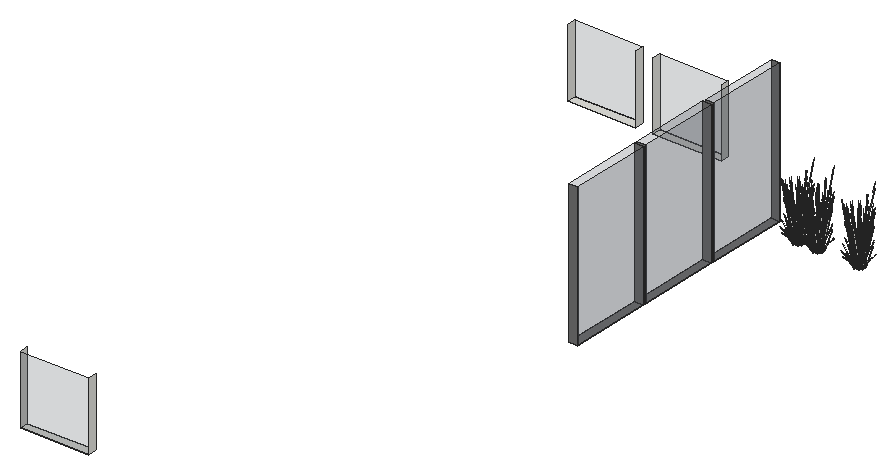
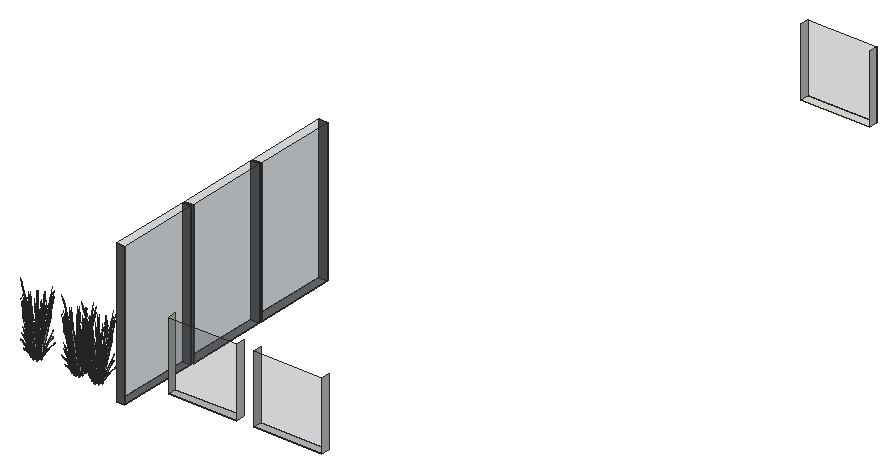
# SketchUp Ruby script. Lengths in inches.
U = 1.inch
M = Sketchup.active_model
def pt(a) = Geom::Point3d.new(a.map { |v| v * U })
def face(e, loops, mat)
  f = e.add_face(loops[0].map { |a| pt(a) })
  loops[1..].each { |l| e.add_face(l.map { |a| pt(a) }).erase! }
  f.material = f.back_material = mat if mat
  f
end
# faces: each face lists its corners as indices into pts; further lists are holes
def faces(e, pts, list, mat = nil) = list.each { |f| face(e, (f[0].is_a?(Array) ? f : [f]).map { |l| l.map { |i| pts[i] } }, mat) }
# xy, xz, yz: faces in a plane at the given z, y or x. An outline is a flat list of corners, or four numbers for a rectangle; further outlines are holes
def ring(l) = l.size == 4 ? [[l[0], l[1]], [l[2], l[1]], [l[2], l[3]], [l[0], l[3]]] : l.each_slice(2).to_a
def flat(e, list, mat, &to3) = list.each { |f| face(e, (f[0].is_a?(Array) ? f : [f]).map { |l| ring(l).map { |u, v| to3.(u, v) } }, mat) }
def xy(e, z, list, mat = nil) = flat(e, list, mat) { |x, y| [x, y, z] }
def xz(e, y, list, mat = nil) = flat(e, list, mat) { |x, z| [x, y, z] }
def yz(e, x, list, mat = nil) = flat(e, list, mat) { |y, z| [x, y, z] }
def lines(e, pts, list) = list.each { |a, b| e.add_line(pt(pts[a]), pt(pts[b])) }
# prism: a flat outline (further loops are holes) pulled along v
def prism(e, loops, v, mat = nil)
  f = face(e, loops, mat); d = Geom::Vector3d.new(v.map { |x| x * U })
  f.pushpull(f.normal.samedirection?(d) ? d.length : -d.length)
end
def box(e, o, s, mat = nil) = prism(e, [[o, [o[0] + s[0], o[1], o[2]], [o[0] + s[0], o[1] + s[1], o[2]], [o[0], o[1] + s[1], o[2]]]], [0, 0, s[2]], mat)
def at(x, y, z, deg = 0) = Geom::Transformation.translation(pt([x, y, z])) * Geom::Transformation.rotation(ORIGIN, Z_AXIS, deg.degrees)
def axes(o, x, y, z) = Geom::Transformation.new([*x, 0, *y, 0, *z, 0, *pt(o).to_a, 1])
def part(name) = M.definitions.add(name)
# library, detail: a bought-in or finely detailed component or shape, given as its bounding box
def library(name, o, s) = part(name).tap { |d| box(d.entities, o, s) }
def detail(e, o, s) = box(e.add_group.entities, o, s)
def put(e, d, t, mat = nil) = e.add_instance(d, t).tap { |i| i.material = mat if mat }
def group(e, t, mat = nil) = e.add_group.tap { |g| g.transformation = t; g.material = mat if mat }.entities
root = M.entities
M.materials.add("Glass_Basic_01").color = [105, 113, 122]
M.materials["Glass_Basic_01"].alpha = 0.25
M.materials.add("LightPink_Translucent").color = [144, 107, 117]
M.materials["LightPink_Translucent"].alpha = 0.75
M.materials.add("M06_Steel_Smoke").color = [114, 114, 114]
c1 = part("blade")
p = [[2.15,0.21,22],[0,0.17,0],[0.09,0.45,0],[2.18,0.31,22],[2.29,0.31,22],[0.38,0.45,0],
  [2.48,0.24,33],[2.49,0.24,33],[2.48,0.22,33]]
faces(c1.entities,p,[[0,1,2,3],[4,5,2,3],[6,3,4,7],[8,0,3,6]])
c2 = part("seeds")
p = [[0.3,-0.1,1.38],[-0.01,-0.03,1.59],[-0.01,-0.03,0.03],[0.14,-0.07,-0.07],[0.29,-0.03,3],[0.15,0.01,3.11]]
faces(c2.entities,p,[[0,1,2,3],[1,0,4,5]],"LightPink_Translucent")
c3 = part("blade with seeds")
put(c3.entities,c1,at(0,0,0))
put(c3.entities,c2,axes([2.4,0.25,30.99],[1.5799,-0.05474,1.17369],[-0.12525,1.92788,0.29478],[-0.07173,-0.02425,1.56792]))
xy(root,655,[[204,295,210,353],[204,355,210,413],[204,415,210,473]],"M06_Steel_Smoke")
xy(root,677.98,[[54,0,102,6]])
xy(root,678,[[60,474,108,480],[120,474,168,480]])
xz(root,0,[[54,677.98,102,725.98]],"Glass_Basic_01")
xz(root,295,[[204,655,210,755]],"M06_Steel_Smoke")
xz(root,353,[[204,655,210,755]],"M06_Steel_Smoke")
xz(root,355,[[204,655,210,755]],"M06_Steel_Smoke")
xz(root,413,[[204,655,210,755]],"M06_Steel_Smoke")
xz(root,415,[[204,655,210,755]],"M06_Steel_Smoke")
xz(root,473,[[204,655,210,755]],"M06_Steel_Smoke")
xz(root,480,[[60,678,108,726],[120,678,168,726]],"Glass_Basic_01")
yz(root,54,[[0,677.98,6,725.98]])
yz(root,60,[[474,678,480,726]])
yz(root,102,[[0,677.98,6,725.98]])
yz(root,108,[[474,678,480,726]])
yz(root,120,[[474,678,480,726]])
yz(root,168,[[474,678,480,726]])
yz(root,204,[[295,655,353,755],[355,655,413,755],[415,655,473,755]],"Glass_Basic_01")
yz(root,210,[[295,655,353,755],[355,655,413,755],[415,655,473,755]],"Glass_Basic_01")
put(root,c3,axes([234.23,462.43,655.03],[0.0269,-0.54769,-0.1216],[0.50939,0.01497,-0.67495],[0.19618,0.03804,1.02557]))
put(root,c3,axes([230.42,460.32,655.03],[0.25281,0.48765,-0.1216],[-0.44869,0.23964,-0.67495],[-0.18908,0.06434,1.02557]))
put(root,c3,axes([234.18,459.26,655.03],[-0.55221,-0.02668,-0.1216],[0.01509,-0.50521,-0.67495],[0.03836,-0.19458,1.02557]))
put(root,c3,axes([234.8,461.41,655.03],[-0.25281,-0.48765,-0.1216],[0.44869,-0.23964,-0.67495],[0.18908,-0.06434,1.02557]))
put(root,c3,axes([232.0625,463.04,655.03],[0.49168,-0.25073,-0.1216],[0.24162,0.44501,-0.67495],[0.06487,0.18753,1.02557]))
put(root,c3,axes([230.99,459.3125,655.03],[-0.0269,0.54769,-0.1216],[-0.50939,-0.01497,-0.67495],[-0.19618,-0.03804,1.02557]))
put(root,c3,axes([233.23,463.02,655.03],[0.2994,-0.46097,-0.1216],[0.43359,0.26557,-0.67495],[0.15072,0.13024,1.02557]))
put(root,c3,axes([230.44,461.48,655.03],[0.46478,0.29695,-0.1216],[-0.26776,0.43004,-0.67495],[-0.13131,0.14949,1.02557]))
put(root,c3,axes([233.16,458.7,655.03],[-0.49168,0.25073,-0.1216],[-0.24162,-0.44501,-0.67495],[-0.06487,-0.18753,1.02557]))
put(root,c3,axes([234.78,460.25,655.03],[-0.46478,-0.29695,-0.1216],[0.26776,-0.43004,-0.67495],[0.13131,-0.14949,1.02557]))
put(root,c3,axes([248.12,462.43,655.03],[0.0269,-0.54769,-0.1216],[0.50939,0.01497,-0.67495],[0.19618,0.03804,1.02557]))
put(root,c3,axes([244.31,460.32,655.03],[0.25281,0.48765,-0.1216],[-0.44869,0.23964,-0.67495],[-0.18908,0.06434,1.02557]))
put(root,c3,axes([248.07,459.26,655.03],[-0.55221,-0.02668,-0.1216],[0.01509,-0.50521,-0.67495],[0.03836,-0.19458,1.02557]))
put(root,c3,axes([248.6875,461.41,655.03],[-0.25281,-0.48765,-0.1216],[0.44869,-0.23964,-0.67495],[0.18908,-0.06434,1.02557]))
put(root,c3,axes([245.95,463.04,655.03],[0.49168,-0.25073,-0.1216],[0.24162,0.44501,-0.67495],[0.06487,0.18753,1.02557]))
put(root,c3,axes([244.88,459.3125,655.03],[-0.0269,0.54769,-0.1216],[-0.50939,-0.01497,-0.67495],[-0.19618,-0.03804,1.02557]))
put(root,c3,axes([247.12,463.02,655.03],[0.2994,-0.46097,-0.1216],[0.43359,0.26557,-0.67495],[0.15072,0.13024,1.02557]))
put(root,c3,axes([244.33,461.48,655.03],[0.46478,0.29695,-0.1216],[-0.26776,0.43004,-0.67495],[-0.13131,0.14949,1.02557]))
put(root,c3,axes([247.05,458.7,655.03],[-0.49168,0.25073,-0.1216],[-0.24162,-0.44501,-0.67495],[-0.06487,-0.18753,1.02557]))
put(root,c3,axes([248.67,460.25,655.03],[-0.46478,-0.29695,-0.1216],[0.26776,-0.43004,-0.67495],[0.13131,-0.14949,1.02557]))
put(root,c3,axes([277.23,462.43,655.03],[0.0269,-0.54769,-0.1216],[0.50939,0.01497,-0.67495],[0.19618,0.03804,1.02557]))
put(root,c3,axes([273.42,460.32,655.03],[0.25281,0.48765,-0.1216],[-0.44869,0.23964,-0.67495],[-0.18908,0.06434,1.02557]))
put(root,c3,axes([277.18,459.26,655.03],[-0.55221,-0.02668,-0.1216],[0.01509,-0.50521,-0.67495],[0.03836,-0.19458,1.02557]))
put(root,c3,axes([277.8,461.41,655.03],[-0.25281,-0.48765,-0.1216],[0.44869,-0.23964,-0.67495],[0.18908,-0.06434,1.02557]))
put(root,c3,axes([275.0625,463.04,655.03],[0.49168,-0.25073,-0.1216],[0.24162,0.44501,-0.67495],[0.06487,0.18753,1.02557]))
put(root,c3,axes([273.99,459.3125,655.03],[-0.0269,0.54769,-0.1216],[-0.50939,-0.01497,-0.67495],[-0.19618,-0.03804,1.02557]))
put(root,c3,axes([276.23,463.02,655.03],[0.2994,-0.46097,-0.1216],[0.43359,0.26557,-0.67495],[0.15072,0.13024,1.02557]))
put(root,c3,axes([273.44,461.48,655.03],[0.46478,0.29695,-0.1216],[-0.26776,0.43004,-0.67495],[-0.13131,0.14949,1.02557]))
put(root,c3,axes([276.16,458.7,655.03],[-0.49168,0.25073,-0.1216],[-0.24162,-0.44501,-0.67495],[-0.06487,-0.18753,1.02557]))
put(root,c3,axes([277.78,460.25,655.03],[-0.46478,-0.29695,-0.1216],[0.26776,-0.43004,-0.67495],[0.13131,-0.14949,1.02557]))
put(root,c3,axes([233.57,460.3,654.47],[-0.43417,-0.27982,1.38283],[0.45844,-0.43566,0.59665],[0.14008,0.26255,1.33663]))
put(root,c3,axes([247.46,460.3,654.47],[-0.43417,-0.27982,1.38283],[0.45844,-0.43566,0.59665],[0.14008,0.26255,1.33663]))
put(root,c3,axes([276.57,460.3,654.47],[-0.43417,-0.27982,1.38283],[0.45844,-0.43566,0.59665],[0.14008,0.26255,1.33663]))
put(root,c3,axes([229.89,460.8125,654.72],[-0.08205,0.06992,1.74944],[0.00698,0.51086,-0.27667],[-0.18807,0.06644,0.14031]))
put(root,c3,axes([236.18,460.65,654.72],[0.06972,-0.08203,1.74944],[-0.08924,-0.50318,-0.27667],[0.17494,-0.0954,0.14031]))
put(root,c3,axes([234.68,462.1,654.72],[0.10779,-0.00911,1.74944],[0.29564,-0.41839,-0.27667],[0.19172,0.05523,0.14031]))
put(root,c3,axes([234.68,458.46,654.72],[-0.00485,-0.10718,1.74944],[-0.40965,-0.30977,-0.27667],[0.06333,-0.18778,0.14031]))
put(root,c3,axes([229.91,462.72,654.72],[-0.01249,0.10657,1.74944],[0.35444,0.37075,-0.27667],[-0.09279,0.17532,0.14031]))
put(root,c3,axes([231.95,464.04,654.72],[0.06369,0.08672,1.74944],[0.51399,0.03407,-0.27667],[0.05169,0.19126,0.14031]))
put(root,c3,axes([232.38,457.53,654.72],[-0.07685,-0.07551,1.74944],[-0.51287,0.04787,-0.27667],[-0.08185,-0.1806,0.14031]))
put(root,c3,axes([230.7,458.36,654.72],[-0.10811,-0.0038,1.74944],[-0.34418,0.38014,-0.27667],[-0.18364,-0.07767,0.14031]))
put(root,c3,axes([243.78,460.8125,654.72],[-0.08205,0.06992,1.74944],[0.00698,0.51086,-0.27667],[-0.18807,0.06644,0.14031]))
put(root,c3,axes([250.0625,460.65,654.72],[0.06972,-0.08203,1.74944],[-0.08924,-0.50318,-0.27667],[0.17494,-0.0954,0.14031]))
put(root,c3,axes([248.5625,462.1,654.72],[0.10779,-0.00911,1.74944],[0.29564,-0.41839,-0.27667],[0.19172,0.05523,0.14031]))
put(root,c3,axes([248.57,458.46,654.72],[-0.00485,-0.10718,1.74944],[-0.40965,-0.30977,-0.27667],[0.06333,-0.18778,0.14031]))
put(root,c3,axes([243.8,462.72,654.72],[-0.01249,0.10657,1.74944],[0.35444,0.37075,-0.27667],[-0.09279,0.17532,0.14031]))
put(root,c3,axes([245.83,464.04,654.72],[0.06369,0.08672,1.74944],[0.51399,0.03407,-0.27667],[0.05169,0.19126,0.14031]))
put(root,c3,axes([246.27,457.53,654.72],[-0.07685,-0.07551,1.74944],[-0.51287,0.04787,-0.27667],[-0.08185,-0.1806,0.14031]))
put(root,c3,axes([244.59,458.36,654.72],[-0.10811,-0.0038,1.74944],[-0.34418,0.38014,-0.27667],[-0.18364,-0.07767,0.14031]))
put(root,c3,axes([272.89,460.8125,654.72],[-0.08205,0.06992,1.74944],[0.00698,0.51086,-0.27667],[-0.18807,0.06644,0.14031]))
put(root,c3,axes([279.18,460.65,654.72],[0.06972,-0.08203,1.74944],[-0.08924,-0.50318,-0.27667],[0.17494,-0.0954,0.14031]))
put(root,c3,axes([277.68,462.1,654.72],[0.10779,-0.00911,1.74944],[0.29564,-0.41839,-0.27667],[0.19172,0.05523,0.14031]))
put(root,c3,axes([277.68,458.46,654.72],[-0.00485,-0.10718,1.74944],[-0.40965,-0.30977,-0.27667],[0.06333,-0.18778,0.14031]))
put(root,c3,axes([272.91,462.72,654.72],[-0.01249,0.10657,1.74944],[0.35444,0.37075,-0.27667],[-0.09279,0.17532,0.14031]))
put(root,c3,axes([274.95,464.04,654.72],[0.06369,0.08672,1.74944],[0.51399,0.03407,-0.27667],[0.05169,0.19126,0.14031]))
put(root,c3,axes([275.38,457.53,654.72],[-0.07685,-0.07551,1.74944],[-0.51287,0.04787,-0.27667],[-0.08185,-0.1806,0.14031]))
put(root,c3,axes([273.7,458.36,654.72],[-0.10811,-0.0038,1.74944],[-0.34418,0.38014,-0.27667],[-0.18364,-0.07767,0.14031]))
put(root,c3,axes([230.28,458.68,654.71],[0.03725,0.05374,1.77383],[-0.17957,0.48312,-0.16761],[-0.18186,0.0035,0.31391]))
put(root,c3,axes([231.86,457.28,654.71],[-0.00937,0.06455,1.77383],[-0.46231,0.23427,-0.16761],[-0.13604,-0.11975,0.31391]))
put(root,c3,axes([232.84,463.4,654.71],[0.00149,-0.0652,1.77383],[0.43058,-0.28766,-0.16761],[0.14956,0.10267,0.31391]))
put(root,c3,axes([228.98,461.33,654.71],[0.06412,0.01444,1.77383],[0.19837,0.47583,-0.16761],[-0.13126,0.12489,0.31391]))
put(root,c3,axes([235.93,460.125,654.71],[-0.06563,-0.00409,1.77383],[-0.27252,-0.43825,-0.16761],[0.10944,-0.1441,0.31391]))
put(root,c3,axes([235.81,462.86,654.71],[-0.04543,-0.04715,1.77383],[0.09938,-0.50538,-0.16761],[0.17896,-0.03229,0.31391]))
put(root,c3,axes([229.87,463.8125,654.71],[0.057,-0.03251,1.77383],[0.47114,0.21627,-0.16761],[-0.01107,0.18007,0.31391]))
put(root,c3,axes([234.58,458.07,654.71],[-0.05103,0.04113,1.77383],[-0.49994,-0.13878,-0.16761],[-0.0181,-0.17951,0.31391]))
put(root,c3,axes([244.17,458.68,654.71],[0.03725,0.05374,1.77383],[-0.17957,0.48312,-0.16761],[-0.18186,0.0035,0.31391]))
put(root,c3,axes([245.74,457.28,654.71],[-0.00937,0.06455,1.77383],[-0.46231,0.23427,-0.16761],[-0.13604,-0.11975,0.31391]))
put(root,c3,axes([246.73,463.4,654.71],[0.00149,-0.0652,1.77383],[0.43058,-0.28766,-0.16761],[0.14956,0.10267,0.31391]))
put(root,c3,axes([242.87,461.33,654.71],[0.06412,0.01444,1.77383],[0.19837,0.47583,-0.16761],[-0.13126,0.12489,0.31391]))
put(root,c3,axes([249.81,460.125,654.71],[-0.06563,-0.00409,1.77383],[-0.27252,-0.43825,-0.16761],[0.10944,-0.1441,0.31391]))
put(root,c3,axes([249.69,462.86,654.71],[-0.04543,-0.04715,1.77383],[0.09938,-0.50538,-0.16761],[0.17896,-0.03229,0.31391]))
put(root,c3,axes([243.76,463.8125,654.71],[0.057,-0.03251,1.77383],[0.47114,0.21627,-0.16761],[-0.01107,0.18007,0.31391]))
put(root,c3,axes([248.46,458.07,654.71],[-0.05103,0.04113,1.77383],[-0.49994,-0.13878,-0.16761],[-0.0181,-0.17951,0.31391]))
put(root,c3,axes([273.28,458.68,654.71],[0.03725,0.05374,1.77383],[-0.17957,0.48312,-0.16761],[-0.18186,0.0035,0.31391]))
put(root,c3,axes([274.86,457.28,654.71],[-0.00937,0.06455,1.77383],[-0.46231,0.23427,-0.16761],[-0.13604,-0.11975,0.31391]))
put(root,c3,axes([275.84,463.4,654.71],[0.00149,-0.0652,1.77383],[0.43058,-0.28766,-0.16761],[0.14956,0.10267,0.31391]))
put(root,c3,axes([271.98,461.33,654.71],[0.06412,0.01444,1.77383],[0.19837,0.47583,-0.16761],[-0.13126,0.12489,0.31391]))
put(root,c3,axes([278.93,460.125,654.71],[-0.06563,-0.00409,1.77383],[-0.27252,-0.43825,-0.16761],[0.10944,-0.1441,0.31391]))
put(root,c3,axes([278.81,462.86,654.71],[-0.04543,-0.04715,1.77383],[0.09938,-0.50538,-0.16761],[0.17896,-0.03229,0.31391]))
put(root,c3,axes([272.87,463.8125,654.71],[0.057,-0.03251,1.77383],[0.47114,0.21627,-0.16761],[-0.01107,0.18007,0.31391]))
put(root,c3,axes([277.58,458.07,654.71],[-0.05103,0.04113,1.77383],[-0.49994,-0.13878,-0.16761],[-0.0181,-0.17951,0.31391]))
put(root,c3,axes([231.04,462.48,655.4],[0.55221,0.02668,-0.13498],[-0.01509,0.50521,-0.74919],[-0.03836,0.19458,1.13838]))
put(root,c3,axes([244.93,462.48,655.4],[0.55221,0.02668,-0.13498],[-0.01509,0.50521,-0.74919],[-0.03836,0.19458,1.13838]))
put(root,c3,axes([274.04,462.48,655.4],[0.55221,0.02668,-0.13498],[-0.01509,0.50521,-0.74919],[-0.03836,0.19458,1.13838]))
put(root,c3,axes([231.98,458.51,655.43],[-0.33533,0.51628,-0.13619],[-0.48563,-0.29744,-0.75594],[-0.16881,-0.14586,1.14864]))
put(root,c3,axes([245.87,458.51,655.43],[-0.33533,0.51628,-0.13619],[-0.48563,-0.29744,-0.75594],[-0.16881,-0.14586,1.14864]))
put(root,c3,axes([274.98,458.51,655.43],[-0.33533,0.51628,-0.13619],[-0.48563,-0.29744,-0.75594],[-0.16881,-0.14586,1.14864]))
put(root,c3,axes([231.88,458.55,654.73],[0.22836,-0.34211,0.0643],[0.3252,0.19918,0.50621],[-0.10513,-0.10968,0.77189]))
put(root,c3,axes([232.07,463.24,654.73],[-0.37023,0.18303,0.0643],[-0.18122,-0.33376,0.50621],[0.03575,0.14712,0.77189]))
put(root,c3,axes([234.95,460.14,654.73],[0.34493,0.22649,0.0643],[-0.20082,0.32253,0.50621],[0.11059,-0.10427,0.77189]))
put(root,c3,axes([235.01,461.4,654.73],[0.18454,0.3672,0.0643],[-0.33652,0.17973,0.50621],[0.14834,-0.03546,0.77189]))
put(root,c3,axes([230.81,459.22,654.73],[0.0253,-0.40952,0.0643],[0.38204,0.01123,0.50621],[-0.14634,-0.04285,0.77189]))
put(root,c3,axes([234.27,459.08,654.73],[0.4129,0.02509,0.0643],[-0.01132,0.37891,0.50621],[0.04321,-0.14514,0.77189]))
put(root,c3,axes([234.42,462.52,654.73],[-0.0253,0.40952,0.0643],[-0.38204,-0.01123,0.50621],[0.14634,0.04285,0.77189]))
put(root,c3,axes([230.27,461.59,654.73],[-0.34493,-0.22649,0.0643],[0.20082,-0.32253,0.50621],[-0.11059,0.10427,0.77189]))
put(root,c3,axes([233.15,458.5,654.73],[0.37023,-0.18303,0.0643],[0.18122,0.33376,0.50621],[-0.03575,-0.14712,0.77189]))
put(root,c3,axes([230.22,460.33,654.73],[-0.18454,-0.3672,0.0643],[0.33652,-0.17973,0.50621],[-0.14834,0.03546,0.77189]))
put(root,c3,axes([233.34,463.19,654.73],[-0.22836,0.34211,0.0643],[-0.3252,-0.19918,0.50621],[0.10513,0.10968,0.77189]))
put(root,c3,axes([230.95,462.66,654.73],[-0.4129,-0.02509,0.0643],[0.01132,-0.37891,0.50621],[-0.04321,0.14514,0.77189]))
put(root,c3,axes([245.77,458.55,654.73],[0.22836,-0.34211,0.0643],[0.3252,0.19918,0.50621],[-0.10513,-0.10968,0.77189]))
put(root,c3,axes([245.96,463.24,654.73],[-0.37023,0.18303,0.0643],[-0.18122,-0.33376,0.50621],[0.03575,0.14712,0.77189]))
put(root,c3,axes([248.84,460.14,654.73],[0.34493,0.22649,0.0643],[-0.20082,0.32253,0.50621],[0.11059,-0.10427,0.77189]))
put(root,c3,axes([248.89,461.4,654.73],[0.18454,0.3672,0.0643],[-0.33652,0.17973,0.50621],[0.14834,-0.03546,0.77189]))
put(root,c3,axes([244.7,459.22,654.73],[0.0253,-0.40952,0.0643],[0.38204,0.01123,0.50621],[-0.14634,-0.04285,0.77189]))
put(root,c3,axes([248.16,459.08,654.73],[0.4129,0.02509,0.0643],[-0.01132,0.37891,0.50621],[0.04321,-0.14514,0.77189]))
put(root,c3,axes([248.3,462.52,654.73],[-0.0253,0.40952,0.0643],[-0.38204,-0.01123,0.50621],[0.14634,0.04285,0.77189]))
put(root,c3,axes([244.16,461.59,654.73],[-0.34493,-0.22649,0.0643],[0.20082,-0.32253,0.50621],[-0.11059,0.10427,0.77189]))
put(root,c3,axes([247.04,458.5,654.73],[0.37023,-0.18303,0.0643],[0.18122,0.33376,0.50621],[-0.03575,-0.14712,0.77189]))
put(root,c3,axes([244.11,460.33,654.73],[-0.18454,-0.3672,0.0643],[0.33652,-0.17973,0.50621],[-0.14834,0.03546,0.77189]))
put(root,c3,axes([247.23,463.19,654.73],[-0.22836,0.34211,0.0643],[-0.3252,-0.19918,0.50621],[0.10513,0.10968,0.77189]))
put(root,c3,axes([244.84,462.66,654.73],[-0.4129,-0.02509,0.0643],[0.01132,-0.37891,0.50621],[-0.04321,0.14514,0.77189]))
put(root,c3,axes([274.88,458.55,654.73],[0.22836,-0.34211,0.0643],[0.3252,0.19918,0.50621],[-0.10513,-0.10968,0.77189]))
put(root,c3,axes([275.07,463.24,654.73],[-0.37023,0.18303,0.0643],[-0.18122,-0.33376,0.50621],[0.03575,0.14712,0.77189]))
put(root,c3,axes([277.95,460.14,654.73],[0.34493,0.22649,0.0643],[-0.20082,0.32253,0.50621],[0.11059,-0.10427,0.77189]))
put(root,c3,axes([278.01,461.4,654.73],[0.18454,0.3672,0.0643],[-0.33652,0.17973,0.50621],[0.14834,-0.03546,0.77189]))
put(root,c3,axes([273.81,459.22,654.73],[0.0253,-0.40952,0.0643],[0.38204,0.01123,0.50621],[-0.14634,-0.04285,0.77189]))
put(root,c3,axes([277.27,459.08,654.73],[0.4129,0.02509,0.0643],[-0.01132,0.37891,0.50621],[0.04321,-0.14514,0.77189]))
put(root,c3,axes([277.42,462.52,654.73],[-0.0253,0.40952,0.0643],[-0.38204,-0.01123,0.50621],[0.14634,0.04285,0.77189]))
put(root,c3,axes([273.27,461.59,654.73],[-0.34493,-0.22649,0.0643],[0.20082,-0.32253,0.50621],[-0.11059,0.10427,0.77189]))
put(root,c3,axes([276.15,458.5,654.73],[0.37023,-0.18303,0.0643],[0.18122,0.33376,0.50621],[-0.03575,-0.14712,0.77189]))
put(root,c3,axes([273.22,460.33,654.73],[-0.18454,-0.3672,0.0643],[0.33652,-0.17973,0.50621],[-0.14834,0.03546,0.77189]))
put(root,c3,axes([276.34,463.19,654.73],[-0.22836,0.34211,0.0643],[-0.3252,-0.19918,0.50621],[0.10513,0.10968,0.77189]))
put(root,c3,axes([273.95,462.66,654.73],[-0.4129,-0.02509,0.0643],[0.01132,-0.37891,0.50621],[-0.04321,0.14514,0.77189]))
put(root,c3,axes([233.02,458.53,654.73],[0.4951,0.14079,0.48003],[-0.1693,0.46287,0.3958],[-0.02975,-0.18203,0.9933]))
put(root,c3,axes([234.45,462.39,654.73],[-0.37048,0.35486,0.48003],[-0.31952,-0.37685,0.3958],[0.17382,0.06546,0.9933]))
put(root,c3,axes([234.97,461.27,654.73],[-0.14195,0.49104,0.48003],[-0.46669,-0.16791,0.3958],[0.18353,-0.02951,0.9933]))
put(root,c3,axes([230.37,461.6875,654.73],[-0.12461,-0.49565,0.48003],[0.48882,-0.08602,0.3958],[-0.14406,0.11657,0.9933]))
put(root,c3,axes([231.08,462.69,654.73],[-0.35779,-0.36745,0.48003],[0.37996,-0.3169,0.3958],[-0.066,0.17239,0.9933]))
put(root,c3,axes([234.14,459.05,654.73],[0.35779,0.36745,0.48003],[-0.37996,0.3169,0.3958],[0.066,-0.17239,0.9933]))
put(root,c3,axes([230.26,460.46,654.73],[0.14195,-0.49104,0.48003],[0.46669,0.16791,0.3958],[-0.18353,0.02951,0.9933]))
put(root,c3,axes([234.86,460.05,654.73],[0.12461,0.49565,0.48003],[-0.48882,0.08602,0.3958],[0.14406,-0.11657,0.9933]))
put(root,c3,axes([233.4375,463.09,654.73],[-0.49974,0.12359,0.48003],[-0.08673,-0.48481,0.3958],[0.11753,0.14288,0.9933]))
put(root,c3,axes([246.91,458.53,654.73],[0.4951,0.14079,0.48003],[-0.1693,0.46287,0.3958],[-0.02975,-0.18203,0.9933]))
put(root,c3,axes([248.34,462.39,654.73],[-0.37048,0.35486,0.48003],[-0.31952,-0.37685,0.3958],[0.17382,0.06546,0.9933]))
put(root,c3,axes([248.86,461.27,654.73],[-0.14195,0.49104,0.48003],[-0.46669,-0.16791,0.3958],[0.18353,-0.02951,0.9933]))
put(root,c3,axes([244.25,461.6875,654.73],[-0.12461,-0.49565,0.48003],[0.48882,-0.08602,0.3958],[-0.14406,0.11657,0.9933]))
put(root,c3,axes([244.97,462.69,654.73],[-0.35779,-0.36745,0.48003],[0.37996,-0.3169,0.3958],[-0.066,0.17239,0.9933]))
put(root,c3,axes([248.03,459.05,654.73],[0.35779,0.36745,0.48003],[-0.37996,0.3169,0.3958],[0.066,-0.17239,0.9933]))
put(root,c3,axes([244.14,460.46,654.73],[0.14195,-0.49104,0.48003],[0.46669,0.16791,0.3958],[-0.18353,0.02951,0.9933]))
put(root,c3,axes([248.74,460.05,654.73],[0.12461,0.49565,0.48003],[-0.48882,0.08602,0.3958],[0.14406,-0.11657,0.9933]))
put(root,c3,axes([247.33,463.09,654.73],[-0.49974,0.12359,0.48003],[-0.08673,-0.48481,0.3958],[0.11753,0.14288,0.9933]))
put(root,c3,axes([276.02,458.53,654.73],[0.4951,0.14079,0.48003],[-0.1693,0.46287,0.3958],[-0.02975,-0.18203,0.9933]))
put(root,c3,axes([277.45,462.39,654.73],[-0.37048,0.35486,0.48003],[-0.31952,-0.37685,0.3958],[0.17382,0.06546,0.9933]))
put(root,c3,axes([277.97,461.27,654.73],[-0.14195,0.49104,0.48003],[-0.46669,-0.16791,0.3958],[0.18353,-0.02951,0.9933]))
put(root,c3,axes([273.37,461.6875,654.73],[-0.12461,-0.49565,0.48003],[0.48882,-0.08602,0.3958],[-0.14406,0.11657,0.9933]))
put(root,c3,axes([274.08,462.69,654.73],[-0.35779,-0.36745,0.48003],[0.37996,-0.3169,0.3958],[-0.066,0.17239,0.9933]))
put(root,c3,axes([277.14,459.05,654.73],[0.35779,0.36745,0.48003],[-0.37996,0.3169,0.3958],[0.066,-0.17239,0.9933]))
put(root,c3,axes([273.26,460.46,654.73],[0.14195,-0.49104,0.48003],[0.46669,0.16791,0.3958],[-0.18353,0.02951,0.9933]))
put(root,c3,axes([277.86,460.05,654.73],[0.12461,0.49565,0.48003],[-0.48882,0.08602,0.3958],[0.14406,-0.11657,0.9933]))
put(root,c3,axes([276.4375,463.09,654.73],[-0.49974,0.12359,0.48003],[-0.08673,-0.48481,0.3958],[0.11753,0.14288,0.9933]))
put(root,c3,axes([232.21,462.87,655.05],[0.15148,-0.41415,0.35414],[0.44193,0.12079,-0.4572],[0.04052,0.16674,0.87481]))
put(root,c3,axes([233.01,458.87,655.05],[-0.15148,0.41415,0.35414],[-0.44193,-0.12079,-0.4572],[-0.04052,-0.16674,0.87481]))
put(root,c3,axes([234.16,462.21,655.05],[-0.28589,-0.33718,0.35414],[0.32644,-0.31919,-0.4572],[0.16586,0.04856,0.87481]))
put(root,c3,axes([234.625,461.27,655.05],[-0.41757,-0.15024,0.35414],[0.12179,-0.4383,-0.4572],[0.16812,-0.04019,0.87481]))
put(root,c3,axes([231.07,459.53,655.05],[0.28589,0.33718,0.35414],[-0.32644,0.31919,-0.4572],[-0.16586,-0.04856,0.87481]))
put(root,c3,axes([231.26,462.4,655.05],[0.33997,-0.28354,0.35414],[0.32182,0.32376,-0.4572],[-0.04897,0.1645,0.87481]))
put(root,c3,axes([230.67,461.52,655.05],[0.43736,-0.07697,0.35414],[0.11549,0.43998,-0.4572],[-0.12533,0.11818,0.87481]))
put(root,c3,axes([233.27,462.8,655.05],[-0.0776,-0.43378,0.35414],[0.44361,-0.11454,-0.4572],[0.11915,0.12431,0.87481]))
put(root,c3,axes([234.56,460.21,655.05],[-0.43736,0.07697,0.35414],[-0.11549,-0.43998,-0.4572],[0.12533,-0.11818,0.87481]))
put(root,c3,axes([230.6,460.47,655.05],[0.41757,0.15024,0.35414],[-0.12179,0.4383,-0.4572],[-0.16812,0.04019,0.87481]))
put(root,c3,axes([233.97,459.34,655.05],[-0.33997,0.28354,0.35414],[-0.32182,-0.32376,-0.4572],[0.04897,-0.1645,0.87481]))
put(root,c3,axes([231.95,458.94,655.05],[0.0776,0.43378,0.35414],[-0.44361,0.11454,-0.4572],[-0.11915,-0.12431,0.87481]))
put(root,c3,axes([246.1,462.87,655.05],[0.15148,-0.41415,0.35414],[0.44193,0.12079,-0.4572],[0.04052,0.16674,0.87481]))
put(root,c3,axes([246.9,458.87,655.05],[-0.15148,0.41415,0.35414],[-0.44193,-0.12079,-0.4572],[-0.04052,-0.16674,0.87481]))
put(root,c3,axes([248.04,462.21,655.05],[-0.28589,-0.33718,0.35414],[0.32644,-0.31919,-0.4572],[0.16586,0.04856,0.87481]))
put(root,c3,axes([248.51,461.27,655.05],[-0.41757,-0.15024,0.35414],[0.12179,-0.4383,-0.4572],[0.16812,-0.04019,0.87481]))
put(root,c3,axes([244.96,459.53,655.05],[0.28589,0.33718,0.35414],[-0.32644,0.31919,-0.4572],[-0.16586,-0.04856,0.87481]))
put(root,c3,axes([245.15,462.4,655.05],[0.33997,-0.28354,0.35414],[0.32182,0.32376,-0.4572],[-0.04897,0.1645,0.87481]))
put(root,c3,axes([244.55,461.52,655.05],[0.43736,-0.07697,0.35414],[0.11549,0.43998,-0.4572],[-0.12533,0.11818,0.87481]))
put(root,c3,axes([247.16,462.8,655.05],[-0.0776,-0.43378,0.35414],[0.44361,-0.11454,-0.4572],[0.11915,0.12431,0.87481]))
put(root,c3,axes([248.44,460.21,655.05],[-0.43736,0.07697,0.35414],[-0.11549,-0.43998,-0.4572],[0.12533,-0.11818,0.87481]))
put(root,c3,axes([244.49,460.47,655.05],[0.41757,0.15024,0.35414],[-0.12179,0.4383,-0.4572],[-0.16812,0.04019,0.87481]))
put(root,c3,axes([247.85,459.34,655.05],[-0.33997,0.28354,0.35414],[-0.32182,-0.32376,-0.4572],[0.04897,-0.1645,0.87481]))
put(root,c3,axes([245.84,458.94,655.05],[0.0776,0.43378,0.35414],[-0.44361,0.11454,-0.4572],[-0.11915,-0.12431,0.87481]))
put(root,c3,axes([275.21,462.87,655.05],[0.15148,-0.41415,0.35414],[0.44193,0.12079,-0.4572],[0.04052,0.16674,0.87481]))
put(root,c3,axes([276.01,458.87,655.05],[-0.15148,0.41415,0.35414],[-0.44193,-0.12079,-0.4572],[-0.04052,-0.16674,0.87481]))
put(root,c3,axes([277.16,462.21,655.05],[-0.28589,-0.33718,0.35414],[0.32644,-0.31919,-0.4572],[0.16586,0.04856,0.87481]))
put(root,c3,axes([277.625,461.27,655.05],[-0.41757,-0.15024,0.35414],[0.12179,-0.4383,-0.4572],[0.16812,-0.04019,0.87481]))
put(root,c3,axes([274.07,459.53,655.05],[0.28589,0.33718,0.35414],[-0.32644,0.31919,-0.4572],[-0.16586,-0.04856,0.87481]))
put(root,c3,axes([274.26,462.4,655.05],[0.33997,-0.28354,0.35414],[0.32182,0.32376,-0.4572],[-0.04897,0.1645,0.87481]))
put(root,c3,axes([273.67,461.52,655.05],[0.43736,-0.07697,0.35414],[0.11549,0.43998,-0.4572],[-0.12533,0.11818,0.87481]))
put(root,c3,axes([276.27,462.8,655.05],[-0.0776,-0.43378,0.35414],[0.44361,-0.11454,-0.4572],[0.11915,0.12431,0.87481]))
put(root,c3,axes([277.56,460.21,655.05],[-0.43736,0.07697,0.35414],[-0.11549,-0.43998,-0.4572],[0.12533,-0.11818,0.87481]))
put(root,c3,axes([273.6,460.47,655.05],[0.41757,0.15024,0.35414],[-0.12179,0.4383,-0.4572],[-0.16812,0.04019,0.87481]))
put(root,c3,axes([276.97,459.34,655.05],[-0.33997,0.28354,0.35414],[-0.32182,-0.32376,-0.4572],[0.04897,-0.1645,0.87481]))
put(root,c3,axes([274.95,458.94,655.05],[0.0776,0.43378,0.35414],[-0.44361,0.11454,-0.4572],[-0.11915,-0.12431,0.87481]))
put(root,c3,axes([232.21,463.21,655.0625],[-0.4951,-0.14079,0.53283],[0.1693,-0.46287,0.43934],[0.02975,0.18203,1.10256]))
put(root,c3,axes([246.09,463.21,655.0625],[-0.4951,-0.14079,0.53283],[0.1693,-0.46287,0.43934],[0.02975,0.18203,1.10256]))
put(root,c3,axes([275.21,463.21,655.0625],[-0.4951,-0.14079,0.53283],[0.1693,-0.46287,0.43934],[0.02975,0.18203,1.10256]))
put(root,c3,axes([230.62,459.22,655.09],[0.41494,-0.39744,0.53763],[0.35786,0.42207,0.4433],[-0.19468,-0.07331,1.11249]))
put(root,c3,axes([231.75,458.43,655.09],[0.55971,-0.13842,0.53763],[0.09714,0.54299,0.4433],[-0.13164,-0.16003,1.11249]))
put(root,c3,axes([244.51,459.22,655.09],[0.41494,-0.39744,0.53763],[0.35786,0.42207,0.4433],[-0.19468,-0.07331,1.11249]))
put(root,c3,axes([245.64,458.43,655.09],[0.55971,-0.13842,0.53763],[0.09714,0.54299,0.4433],[-0.13164,-0.16003,1.11249]))
put(root,c3,axes([273.62,459.22,655.09],[0.41494,-0.39744,0.53763],[0.35786,0.42207,0.4433],[-0.19468,-0.07331,1.11249]))
put(root,c3,axes([274.75,458.43,655.09],[0.55971,-0.13842,0.53763],[0.09714,0.54299,0.4433],[-0.13164,-0.16003,1.11249]))
put(root,c3,axes([232.81,464.34,655.65],[0.34721,-0.30895,-0.06488],[0.31814,0.33837,-0.29416],[0.0224,0.09588,0.97024]))
put(root,c3,axes([229.68,462.77,655.65],[0.44338,0.14375,-0.06488],[-0.13639,0.44245,-0.29416],[-0.07252,0.06718,0.97024]))
put(root,c3,axes([246.69,464.34,655.65],[0.34721,-0.30895,-0.06488],[0.31814,0.33837,-0.29416],[0.0224,0.09588,0.97024]))
put(root,c3,axes([243.5625,462.77,655.65],[0.44338,0.14375,-0.06488],[-0.13639,0.44245,-0.29416],[-0.07252,0.06718,0.97024]))
put(root,c3,axes([275.81,464.34,655.65],[0.34721,-0.30895,-0.06488],[0.31814,0.33837,-0.29416],[0.0224,0.09588,0.97024]))
put(root,c3,axes([272.68,462.77,655.65],[0.44338,0.14375,-0.06488],[-0.13639,0.44245,-0.29416],[-0.07252,0.06718,0.97024]))
